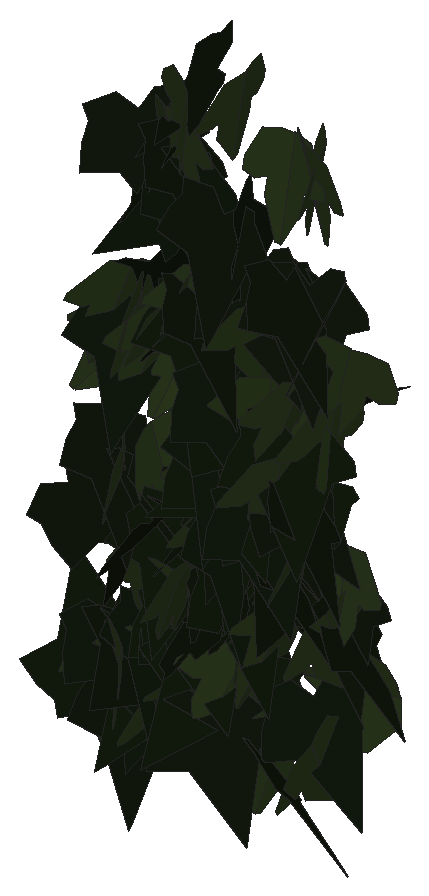
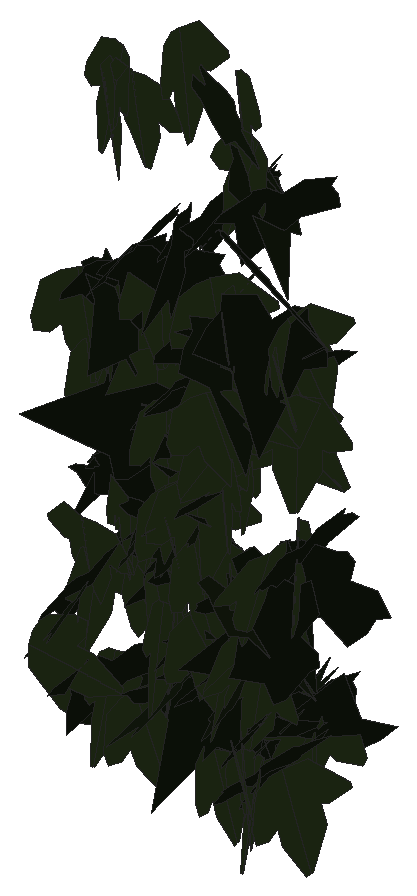
# SketchUp Ruby script. Lengths in inches.
U = 1.inch
M = Sketchup.active_model
def pt(a) = Geom::Point3d.new(a.map { |v| v * U })
def face(e, loops, mat)
  f = e.add_face(loops[0].map { |a| pt(a) })
  loops[1..].each { |l| e.add_face(l.map { |a| pt(a) }).erase! }
  f.material = f.back_material = mat if mat
  f
end
# faces: each face lists its corners as indices into pts; further lists are holes
def faces(e, pts, list, mat = nil) = list.each { |f| face(e, (f[0].is_a?(Array) ? f : [f]).map { |l| l.map { |i| pts[i] } }, mat) }
# xy, xz, yz: faces in a plane at the given z, y or x. An outline is a flat list of corners, or four numbers for a rectangle; further outlines are holes
def ring(l) = l.size == 4 ? [[l[0], l[1]], [l[2], l[1]], [l[2], l[3]], [l[0], l[3]]] : l.each_slice(2).to_a
def flat(e, list, mat, &to3) = list.each { |f| face(e, (f[0].is_a?(Array) ? f : [f]).map { |l| ring(l).map { |u, v| to3.(u, v) } }, mat) }
def xy(e, z, list, mat = nil) = flat(e, list, mat) { |x, y| [x, y, z] }
def xz(e, y, list, mat = nil) = flat(e, list, mat) { |x, z| [x, y, z] }
def yz(e, x, list, mat = nil) = flat(e, list, mat) { |y, z| [x, y, z] }
def lines(e, pts, list) = list.each { |a, b| e.add_line(pt(pts[a]), pt(pts[b])) }
# prism: a flat outline (further loops are holes) pulled along v
def prism(e, loops, v, mat = nil)
  f = face(e, loops, mat); d = Geom::Vector3d.new(v.map { |x| x * U })
  f.pushpull(f.normal.samedirection?(d) ? d.length : -d.length)
end
def box(e, o, s, mat = nil) = prism(e, [[o, [o[0] + s[0], o[1], o[2]], [o[0] + s[0], o[1] + s[1], o[2]], [o[0], o[1] + s[1], o[2]]]], [0, 0, s[2]], mat)
def at(x, y, z, deg = 0) = Geom::Transformation.translation(pt([x, y, z])) * Geom::Transformation.rotation(ORIGIN, Z_AXIS, deg.degrees)
def axes(o, x, y, z) = Geom::Transformation.new([*x, 0, *y, 0, *z, 0, *pt(o).to_a, 1])
def part(name) = M.definitions.add(name)
# library, detail: a bought-in or finely detailed component or shape, given as its bounding box
def library(name, o, s) = part(name).tap { |d| box(d.entities, o, s) }
def detail(e, o, s) = box(e.add_group.entities, o, s)
def put(e, d, t, mat = nil) = e.add_instance(d, t).tap { |i| i.material = mat if mat }
def group(e, t, mat = nil) = e.add_group.tap { |g| g.transformation = t; g.material = mat if mat }.entities
root = M.entities
M.materials.add("efeu1").color = [18, 25, 13]
M.materials.add("efeu2").color = [43, 57, 29]
c1 = part("ivyleaf_9")
p = [[1.54,2.16,1.25],[1.36,2.04,1.19],[-0.21,0.99,0.68],[-0.71,1.11,0.82],[-0.85,0.86,0.67],[-0.8,0.17,0.21],
  [-0.9,-0.01,0.1],[-0.67,-0.16,-0.02],[-0.08,-0.08,-0.05],[-0.03,-0.6,-0.4],[0.65,-0.88,-0.66],[0.83,-0.6,-0.49],
  [1.29,-0.42,-0.43],[1.8125,-0.07,-0.26],[1.21,0.44,0.15]]
faces(c1.entities,p,[[0,1,2,3,4,5,6,7,8,9,10,11,12,13,14]],"efeu1")
c2 = part("ivyleaf_10")
p = [[0,0.5,-0.03],[-0.0625,2.02,-0.43],[-0.19,2.01,-0.46],[-0.54,1.05,-0.29],[-0.52,0.625,-0.18],[-0.83,0.76,-0.28],
  [-1.16,0.64,-0.33],[-1.15,0.33,-0.24],[-0.77,-0.39,0.02],[-0.3,-0.51,0.16],[0.04,-0.48,0.23],[-0.02,2.01,-0.4375],
  [-0.06,2.01,-0.43],[0.04,-0.49,0.23],[0.67,-0.49,0.14],[1.38,0.36,-0.2],[1.375,0.51,-0.24],[0.81,0.65,-0.19],
  [0.62,0.59,-0.15],[0.6,1.09,-0.28],[0.5,1.23,-0.31]]
faces(c2.entities,p,[[0,1,2,3,4,5,6,7,8,9,10],[11,12,0,13,14,15,16,17,18,19,20]],"efeu2")
put(root,c1,axes([29.55,222.72,237.39],[-0.11068,-0.47885,0.09193],[-0.00408,-0.09335,-0.49119],[0.48758,-0.10948,0.01676]))
put(root,c1,axes([29.4,222.7,240.04],[-0.02743,-0.49108,0.08995],[-0.00472,-0.08983,-0.49184],[0.49922,-0.02783,0.00029]))
put(root,c2,axes([30.36,222.42,237.46],[-0.15306,-0.47509,-0.02927],[-0.00052,0.03092,-0.49904],[0.47599,-0.15274,-0.00996]))
put(root,c1,axes([29.6,222.53,237.38],[-0.10075,-0.40992,-0.26798],[0.22774,0.203,-0.39614],[0.43357,-0.20188,0.1458]))
put(root,c1,axes([28.26,222.69,238.41],[-0.12158,-0.48391,0.03236],[-0.00094,-0.03313,-0.4989],[0.48499,-0.12137,0.00714]))
put(root,c1,axes([29.46,222.47,234.18],[-0.10537,-0.39892,-0.28241],[0.07367,0.27264,-0.4126],[0.48319,-0.12856,0.00132]))
put(root,c2,axes([29.125,222.32,241.5],[0.32194,-0.29984,-0.23758],[-0.09758,0.23588,-0.42993],[0.3699,0.32319,0.09336]))
put(root,c1,axes([30.19,222.49,233.82],[0.38743,-0.30001,0.09949],[0.08008,-0.05907,-0.49],[0.30576,0.39561,0.00228]))
put(root,c1,axes([30.11,222.51,236.92],[-0.01543,-0.45455,-0.20772],[-0.00937,0.20805,-0.45456],[0.49967,-0.01013,-0.01493]))
put(root,c1,axes([29.25,222.82,234.46],[-0.26958,-0.37371,0.19409],[-0.03615,-0.20906,-0.45275],[0.41955,-0.25814,0.0857]))
put(root,c2,axes([28.125,222.61,238.91],[-0.07709,-0.46601,0.16399],[-0.00712,-0.1649,-0.47197],[0.49397,-0.0751,0.01879]))
put(root,c2,axes([28.56,222.68,238.46],[-0.04941,-0.44936,0.21362],[0.02303,-0.2165,-0.45011],[0.49702,-0.03464,0.0421]))
put(root,c1,axes([30.39,222.65,237.7],[-0.24399,-0.35765,-0.25011],[0.2335,0.1351,-0.42098],[0.36871,-0.32224,0.10109]))
put(root,c2,axes([29.8,222.5,241.875],[0.01906,-0.49624,-0.05812],[0.00952,0.05851,-0.49647],[0.49955,0.01782,0.01168]))
put(root,c1,axes([30.07,222.75,237.26],[-0.44642,-0.06386,0.21594],[-0.19715,-0.12086,-0.44331],[0.10881,-0.48095,0.08273]))
put(root,c1,axes([30.06,222.89,235.94],[0.00131,-0.36834,0.33812],[0.02178,-0.33776,-0.36803],[0.49952,0.0157,0.01516]))
put(root,c1,axes([28.11,222.92,234.22],[-0.14597,-0.29232,0.37847],[0.0317,-0.40075,-0.29731],[0.47717,-0.0628,0.13553]))
put(root,c2,axes([30.4,222.55,241.23],[0.49191,-0.08827,0.0154],[0.02397,0.0468,-0.49723],[0.08634,0.48992,0.05028]))
put(root,c1,axes([29.12,222.69,238.95],[0.17978,-0.46538,0.03313],[0.02568,-0.02558,-0.49868],[0.46585,0.18101,0.0147]))
put(root,c2,axes([28.17,222.41,234.42],[0.31343,-0.30558,-0.24163],[-0.10118,0.23563,-0.42924],[0.3762,0.31797,0.08587]))
put(root,c2,axes([28.92,222.6,235.6],[0.09995,-0.48987,0.0058],[0.00141,-0.00563,-0.49997],[0.48991,0.09996,0.00026]))
put(root,c1,axes([30.43,222.7,237.01],[0.23241,-0.43616,0.07587],[0.03256,-0.06862,-0.4942],[0.44151,0.23465,-0.00349]))
put(root,c2,axes([29.57,222.77,234.72],[-0.19971,-0.38001,0.25634],[-0.01038,-0.27579,-0.41693],[0.45827,-0.17185,0.10227]))
put(root,c2,axes([30.8,222.47,241.32],[-0.42472,0.2617,0.03357],[-0.04493,-0.00906,-0.49789],[-0.25999,-0.42595,0.03122]))
put(root,c2,axes([30.09,222.8,235.38],[0.00929,-0.42907,0.25653],[0.01808,-0.25612,-0.42904],[0.49959,0.01725,0.01076]))
put(root,c1,axes([29.48,222.82,236.17],[0.06401,-0.49176,0.06386],[0.00625,-0.06359,-0.4959],[0.49585,0.06428,-0.00199]))
put(root,c1,axes([28.88,222.76,240.38],[0.12427,-0.4826,-0.04069],[-0.0058,0.04053,-0.49832],[0.48428,0.12432,0.00447]))
put(root,c1,axes([28.06,222.85,233.74],[-0.01033,-0.49969,0.01434],[0.00246,-0.01439,-0.49979],[0.49989,-0.01026,0.00276]))
put(root,c2,axes([30.29,222.77,238.15],[-0.01573,-0.47689,0.14944],[-0.01098,-0.14914,-0.47711],[0.49963,-0.01829,-0.00578]))
put(root,c1,axes([29.34,222.25,235.04],[0.14222,0.26786,0.39752],[-0.13842,0.41993,-0.23344],[-0.45892,-0.04365,0.19361]))
put(root,c1,axes([29.6,222.8,235.68],[0.04975,-0.48748,-0.09942],[0.01383,0.10123,-0.48945],[0.49733,0.04595,0.02355]))
put(root,c1,axes([29.4,222.73,238.01],[0.05488,-0.46366,-0.1789],[0.00404,0.1804,-0.4663],[0.49696,0.04973,0.02355]))
put(root,c2,axes([29.98,222.68,239.08],[-0.1988,-0.45785,-0.02923],[0.00471,0.02982,-0.49909],[0.45875,-0.19872,-0.00755]))
put(root,c1,axes([27.89,222.6,234],[-0.43456,-0.20874,0.13261],[0.11724,0.06217,0.48207],[-0.21775,0.45007,-0.00508]))
put(root,c1,axes([28.77,222.43,240.5625],[-0.17975,0.43479,0.16926],[-0.05494,0.1604,-0.47038],[-0.46333,-0.18769,-0.00989]))
put(root,c1,axes([30.2,222.8125,239.46],[0.16104,-0.46995,-0.05668],[0.00227,0.06064,-0.4963],[0.47335,0.15959,0.02166]))
put(root,c2,axes([28.37,222.58,238.59],[0.09927,-0.43921,-0.21734],[0.02393,0.22584,-0.44545],[0.48946,0.07804,0.06586]))
put(root,c2,axes([28.95,222.625,235.63],[0.17043,-0.43629,-0.17494],[-0.03515,0.17373,-0.46753],[0.46874,0.17166,0.02854]))
put(root,c1,axes([29.76,222.59,235.73],[-0.35733,0.31956,0.14212],[-0.09576,0.10602,-0.47916],[-0.33637,-0.36965,-0.01456]))
put(root,c2,axes([30.58,222.78,237.71],[0.41531,-0.27683,0.02965],[0.02636,-0.0139,-0.49911],[0.27717,0.41614,0.00305]))
put(root,c2,axes([30.68,222.71,241.2],[0.24292,-0.4304,-0.07578],[-0.00266,0.08525,-0.49267],[0.43701,0.23976,0.03913]))
put(root,c1,axes([29.97,222.79,236.26],[0.32673,-0.37844,-0.00519],[-0.00101,0.00598,-0.49996],[0.37848,0.32672,0.00314]))
put(root,c2,axes([28.77,222.6875,240.96],[-0.44131,0.22196,-0.07736],[0.0575,-0.05763,-0.49333],[-0.22791,-0.44431,0.02534]))
put(root,c2,axes([27.87,222.63,234.27],[-0.33879,-0.30334,-0.20785],[0.17996,0.10969,-0.45341],[0.32068,-0.38204,0.03486]))
put(root,c2,axes([29.13,222.82,239.125],[-0.26472,-0.4177,0.07386],[0.01642,-0.09709,-0.49021],[0.42386,-0.25711,0.06512]))
put(root,c1,axes([29.52,222.73,237.79],[0.11417,-0.41348,-0.2569],[-0.00655,0.26254,-0.42548],[0.48675,0.10052,0.05453]))
put(root,c1,axes([29.08,222.91,238.75],[-0.20656,-0.42713,-0.15778],[0.06728,0.14272,-0.47445],[0.45034,-0.21723,-0.00148]))
put(root,c1,axes([28.41,222.6875,235.99],[-0.1688,0.44237,-0.16068],[0.05999,-0.14908,-0.47347],[-0.46681,-0.17912,-0.00275]))
put(root,c1,axes([29.2,222.8,241.71],[-0.41582,0.25794,-0.10277],[0.07297,-0.07705,-0.48861],[-0.2679,-0.42134,0.02643]))
put(root,c1,axes([27.84,222.79,234.61],[0.07959,-0.43637,-0.23076],[0.01208,0.23539,-0.44096],[0.49348,0.06461,0.04801]))
put(root,c1,axes([28.67,222.88,240.6],[0.20956,-0.45328,-0.02484],[0.00622,0.03022,-0.49905],[0.45392,0.20886,0.0183]))
put(root,c2,axes([28.87,222.82,239.04],[0.17812,-0.46669,-0.02169],[0.00411,0.02477,-0.49937],[0.46718,0.17772,0.01266]))
put(root,c1,axes([27.43,222.65,236.15],[0.12002,-0.1084,-0.47312],[0.29566,0.40285,-0.0173],[0.38494,-0.27561,0.1608]))
put(root,c1,axes([28.86,222.94,235.09],[-0.09597,-0.44339,-0.21023],[0.22452,0.15079,-0.42054],[0.43632,-0.17512,0.17016]))
put(root,c2,axes([28.0625,222.94,238.66],[0.27813,-0.39773,0.12024],[0.07445,-0.09465,-0.48528],[0.40878,0.28785,0.00657]))
put(root,c1,axes([28.16,222.86,240.8],[-0.02038,-0.43993,-0.23673],[0.0761,0.23143,-0.43663],[0.49375,-0.05382,0.05753]))
put(root,c1,axes([29.78,222.83,239.4],[-0.12027,-0.36384,-0.32118],[0.1394,0.29106,-0.38191],[0.46487,-0.18141,0.03142]))
put(root,c2,axes([30.39,222.78,236.38],[0.12898,-0.46782,-0.12046],[-0.01485,0.12078,-0.48496],[0.48285,0.12868,0.01726]))
put(root,c2,axes([28.6,222.74,238.65],[0.01584,-0.46832,-0.17444],[-0.00899,0.17423,-0.46857],[0.49967,0.01798,-0.0029]))
put(root,c2,axes([28.33,222.78,235.37],[-0.49772,0.04586,0.01326],[-0.01415,-0.00905,-0.49972],[-0.04559,-0.49781,0.01031]))
put(root,c2,axes([29.89,222.88,238.02],[-0.33704,-0.36898,0.01606],[0.01553,-0.03588,-0.49847],[0.369,-0.33551,0.03565]))
put(root,c1,axes([28.33,223.19,234.11],[-0.32389,-0.36802,0.09828],[-0.03102,-0.10309,-0.48827],[0.37965,-0.32239,0.04395]))
put(root,c1,axes([27.68,223.08,236.68],[0.04733,-0.4975,-0.01589],[-0.01108,0.01491,-0.49965],[0.49763,0.04765,-0.00962]))
put(root,c2,axes([28.8,222.98,238.35],[0.33293,0.30951,-0.20822],[-0.15759,-0.13627,-0.45453],[-0.33811,0.36828,0.00682]))
put(root,c1,axes([30.28,223.07,239.32],[-0.0828,-0.48214,-0.10338],[0.0288,0.09992,-0.48907],[0.49225,-0.08695,0.01122]))
put(root,c2,axes([30.25,222.87,236.53],[0.02051,-0.48777,-0.108],[0.00044,0.10811,-0.48817],[0.49958,0.01993,0.00487]))
put(root,c2,axes([28.55,223.06,237.375],[-0.27156,0.21005,-0.3635],[0.21888,-0.29859,-0.33606],[-0.35825,-0.34165,0.07021]))
put(root,c1,axes([30.16,222.81,237.11],[0.18577,-0.35035,-0.30454],[-0.06216,0.3063,-0.39028],[0.46003,0.18286,0.07025]))
put(root,c2,axes([30.67,222.93,237.92],[-0.0825,-0.49255,-0.0242],[0.00567,0.02359,-0.49941],[0.49311,-0.08267,0.0017]))
put(root,c1,axes([28.55,223.17,235.8],[-0.20909,-0.45412,-0.00759],[0.02349,-0.00247,-0.49944],[0.45357,-0.20921,0.02237]))
put(root,c1,axes([29.54,223.16,236.48],[-0.36175,-0.2866,-0.19235],[0.22599,0.01395,-0.4458],[0.2609,-0.40947,0.11944]))
put(root,c2,axes([29.08,223,234.92],[0.12972,-0.48259,0.01679],[0.00487,-0.01608,-0.49972],[0.48286,0.12981,0.00053]))
put(root,c2,axes([30.57,222.77,233.96],[-0.01476,-0.42462,-0.26359],[0.02213,0.26289,-0.42474],[0.49929,-0.0242,0.01103]))
put(root,c1,axes([28.12,223.22,234.41],[0.01982,-0.48076,0.13594],[0.01908,-0.13522,-0.48099],[0.49924,0.02425,0.01299]))
put(root,c2,axes([28.48,222.9,233.87],[-0.04157,-0.48624,-0.10881],[0.01932,0.10753,-0.48792],[0.49789,-0.04477,0.00985]))
put(root,c1,axes([28.68,222.98,240],[-0.46274,0.18318,0.04813],[-0.04612,0.01427,-0.49766],[-0.1837,-0.46502,0.00369]))
put(root,c2,axes([28.02,223.03,238.07],[0.34606,0.15447,-0.32616],[-0.32419,-0.06547,-0.37498],[-0.15856,0.47101,0.05484]))
put(root,c2,axes([29.75,222.99,235.46],[0.12187,-0.48423,-0.02594],[-0.00131,0.02642,-0.4993],[0.48492,0.12176,0.00517]))
put(root,c2,axes([30.9,222.97,238.7],[-0.44911,-0.16788,0.14184],[-0.12356,-0.074,-0.47881],[0.18175,-0.46513,0.02498]))
put(root,c1,axes([28.66,223.07,234.85],[0.08898,-0.47712,-0.12015],[0.04214,0.12904,-0.48122],[0.49021,0.07551,0.06317]))
put(root,c1,axes([29.29,223.29,236.54],[-0.15682,-0.45962,0.11897],[-0.00006,-0.12527,-0.48405],[0.47477,-0.15183,0.03924]))
put(root,c2,axes([29.91,223.1,233.85],[-0.22213,-0.42366,0.14549],[-0.02655,-0.14966,-0.47634],[0.44716,-0.21934,0.04399]))
put(root,c2,axes([28.87,222.96,237.27],[0.35913,-0.34248,-0.06107],[0.02505,0.11301,-0.48642],[0.34698,0.34632,0.09833]))
put(root,c2,axes([27.91,222.94,238.13],[-0.47374,-0.14248,0.07262],[-0.07332,-0.00825,-0.49453],[0.14212,-0.4792,-0.01308]))
put(root,c1,axes([29.45,223.35,234.47],[-0.35366,-0.30467,0.17917],[-0.05125,-0.20658,-0.45244],[0.34971,-0.33839,0.11489]))
put(root,c1,axes([28.36,222.8,239.1],[0.18535,0.44868,-0.11971],[-0.04943,-0.1091,-0.48544],[-0.46174,0.19178,0.00391]))
put(root,c2,axes([29.59,223.07,236.27],[0.35062,-0.27301,0.2292],[0.27673,0.00583,-0.4164],[0.22469,0.41885,0.15518]))
put(root,c1,axes([29.26,223.06,236.51],[0.37912,-0.30904,0.10373],[0.10843,-0.0305,-0.48715],[0.30743,0.39187,0.04389]))
put(root,c2,axes([27.875,222.87,236.58],[0.17589,-0.38094,-0.27193],[-0.03621,0.27855,-0.41364],[0.46664,0.1652,0.0704]))
put(root,c2,axes([29.6,223.04,237.56],[-0.14353,-0.47654,-0.04803],[0.01353,0.04609,-0.49769],[0.47877,-0.14416,-0.00034]))
put(root,c1,axes([29.08,223.1,235.32],[0.20497,-0.43299,-0.14319],[-0.06436,0.12796,-0.47905],[0.45149,0.21482,-0.00328]))
put(root,c1,axes([28.875,222.83,238.65],[-0.067,0.49447,0.03186],[-0.03047,0.02798,-0.49829],[-0.49455,-0.06871,0.02638]))
put(root,c1,axes([30.31,223.125,234.34],[0.0432,-0.44569,-0.22246],[0.03701,0.22555,-0.4447],[0.49675,0.02196,0.05248]))
put(root,c2,axes([30.59,222.99,235.42],[-0.04641,-0.46622,-0.17461],[0.06011,0.16884,-0.46678],[0.4942,-0.06432,0.04038]))
put(root,c1,axes([30.23,223.33,236.88],[-0.46484,-0.15489,0.09966],[-0.088,-0.0509,-0.48956],[0.1618,-0.47267,0.02006]))
put(root,c2,axes([27.76,223.23,233.67],[-0.17459,-0.45428,0.11466],[-0.00244,-0.12148,-0.48501],[0.46852,-0.16991,0.0402]))
put(root,c2,axes([28.76,223.06,237.68],[-0.44496,-0.00771,-0.22793],[0.22787,0.00541,-0.44502],[0.00933,-0.49991,-0.0013]))
put(root,c1,axes([28.01,223.46,233.92],[-0.14576,-0.4575,0.13944],[0.03281,-0.15499,-0.47424],[0.47715,-0.1291,0.07521]))
put(root,c2,axes([29.4,223.27,236.51],[0.29653,-0.39604,0.07223],[0.06235,-0.04344,-0.49419],[0.39772,0.3021,0.02363]))
put(root,c2,axes([29.1,223.18,236.78],[-0.35502,-0.35002,0.03812],[-0.0256,-0.02833,-0.49854],[0.35115,-0.35593,0.00219]))
put(root,c2,axes([29.35,223.28,236.67],[-0.17991,-0.45438,0.10568],[0.00232,-0.11414,-0.48679],[0.4665,-0.17467,0.04317]))
put(root,c1,axes([29.55,222.82,239.74],[0.04777,0.15691,-0.47233],[-0.4135,0.2766,0.05007],[0.27701,0.38584,0.15619]))
put(root,c2,axes([29.46,223.04,235.11],[0.21267,-0.38116,-0.2439],[-0.00728,0.26658,-0.42294],[0.45246,0.18344,0.10783]))
put(root,c2,axes([30.53,223.26,235.96],[0.49362,-0.04537,0.06542],[0.06506,-0.00687,-0.4957],[0.04588,0.49789,-0.00088]))
put(root,c2,axes([28.73,223.36,238.09],[-0.41566,-0.227,0.16031],[-0.04941,-0.22348,-0.44454],[0.27348,-0.38539,0.16335]))
put(root,c2,axes([28.96,223.27,236.12],[-0.0775,-0.49388,0.00854],[-0.00902,-0.00723,-0.49987],[0.49388,-0.07763,-0.00779]))
put(root,c1,axes([28.5625,223.21,235.84],[-0.35207,0.35503,-0.00128],[-0.06938,-0.07057,-0.49011],[-0.34819,-0.34493,0.09895]))
put(root,c1,axes([28.27,223.41,234.9375],[0.25429,-0.41834,0.10164],[0.05279,-0.08686,-0.48956],[0.42726,0.25971,-0.00001]))
put(root,c1,axes([30.4,222.86,238.65],[-0.00585,0.30789,0.39391],[0.00946,0.39394,-0.30777],[-0.49988,0.00386,-0.01043]))
put(root,c2,axes([28.12,223.32,235.06],[-0.49384,0.05539,-0.05523],[0.04039,-0.12181,-0.48325],[-0.06699,-0.48176,0.11584]))
put(root,c2,axes([28.8,223.39,235.35],[-0.24109,-0.4249,0.10648],[-0.01491,-0.11351,-0.48672],[0.43778,-0.23786,0.04206]))
put(root,c1,axes([30.34,223.47,235.61],[0.09125,-0.48995,-0.04026],[0.00127,0.04118,-0.4983],[0.4916,0.09084,0.00877]))
put(root,c1,axes([30.52,223.34,235.34],[0.31042,-0.37788,-0.10413],[-0.0616,0.08415,-0.489],[0.3871,0.31642,0.00569]))
put(root,c2,axes([28.3125,223.26,233.95],[0.19791,-0.42883,-0.16412],[-0.02922,0.16659,-0.47052],[0.45824,0.19583,0.04088]))
put(root,c2,axes([28.27,223.42,233.97],[0.27277,-0.41751,0.03576],[0.02731,-0.02487,-0.49863],[0.41815,0.27398,0.00924]))
put(root,c2,axes([28.5625,223.44,233.87],[0.005,-0.49497,0.07053],[0.02747,-0.07016,-0.49429],[0.49922,0.00882,0.02649]))
put(root,c1,axes([27.64,223.26,235.66],[0.44453,-0.0517,0.22299],[0.22156,-0.02514,-0.44752],[0.05749,0.49668,0.00056]))
put(root,c1,axes([29.77,223.13,237.55],[0.29975,0.006,0.40014],[0.33802,0.26384,-0.25716],[-0.21423,0.42468,0.15412]))
put(root,c2,axes([28.2,223.27,233.68],[-0.32279,0.33459,0.18401],[-0.14639,0.11411,-0.46427],[-0.35267,-0.3536,0.0243]))
put(root,c2,axes([29.45,223.29,235.18],[0.03713,-0.41217,-0.2806],[-0.02599,0.2794,-0.41384],[0.49794,0.04531,-0.00068]))
put(root,c1,axes([28.77,223.29,234.57],[0.46256,0.085,-0.16975],[-0.1738,0.00968,-0.46872],[-0.0764,0.49263,0.0385]))
put(root,c2,axes([28.45,223.38,235.29],[0.19037,-0.40824,-0.21701],[0.05262,0.25229,-0.42846],[0.45934,0.1403,0.13902]))
put(root,c1,axes([29.04,223.54,234.6875],[0.29585,-0.3905,-0.09992],[0.00903,0.13033,-0.48263],[0.40298,0.28376,0.08416]))
put(root,c2,axes([27.96,223.44,236.48],[-0.01007,0.49818,0.04138],[0.0029,0.04144,-0.49827],[-0.49989,-0.00979,-0.00372]))
put(root,c2,axes([30.85,223.51,234.46],[0.08249,-0.01119,-0.49302],[-0.47716,0.12443,-0.08266],[0.12454,0.48414,0.00985]))
put(root,c2,axes([28.37,223.21,235.23],[0.00676,-0.00599,0.49992],[-0.2073,0.45493,0.00826],[-0.45495,-0.20737,0.00366]))
